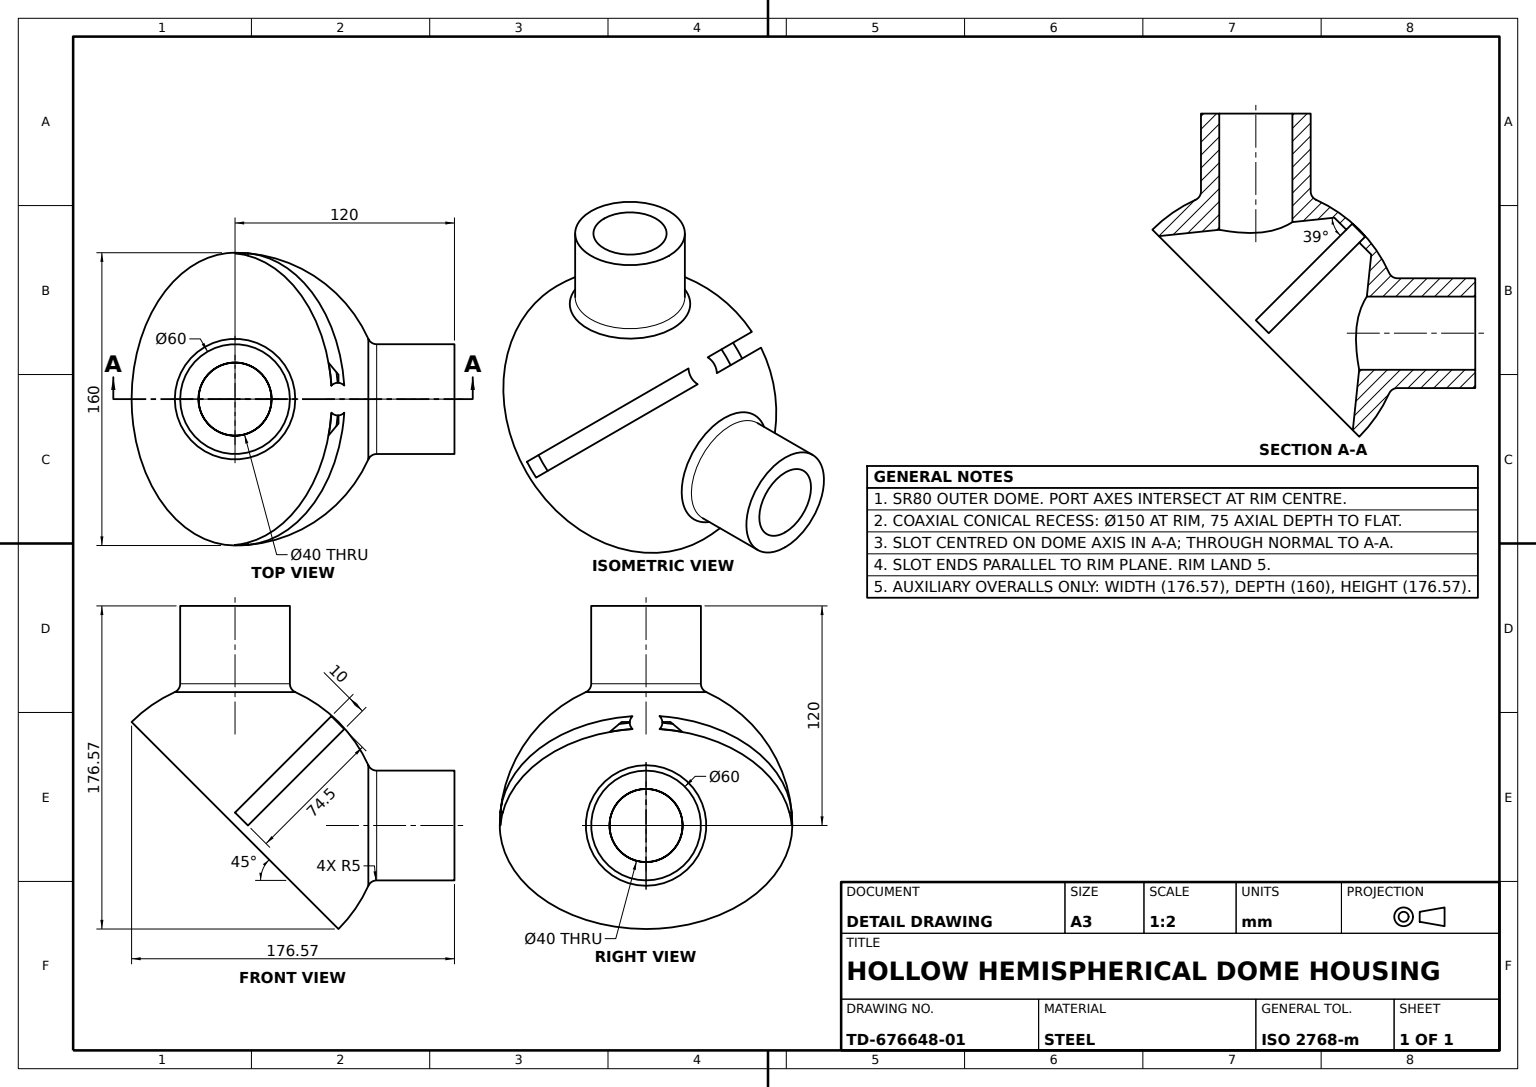
ISO-10303-21;
HEADER;
FILE_DESCRIPTION((''),'2;1');
FILE_NAME('','',(''),(''),'','','');
FILE_SCHEMA(('AUTOMOTIVE_DESIGN'));
ENDSEC;
DATA;
#1=APPLICATION_CONTEXT('');
#2=PRODUCT_CONTEXT('',#1,'mechanical');
#3=PRODUCT('','','',(#2));
#4=PRODUCT_DEFINITION_FORMATION('','',#3);
#5=PRODUCT_DEFINITION_CONTEXT('',#1,'design');
#6=PRODUCT_DEFINITION('','',#4,#5);
#7=PRODUCT_DEFINITION_SHAPE('','',#6);
#8=(LENGTH_UNIT()NAMED_UNIT(*)SI_UNIT(.MILLI.,.METRE.));
#9=(NAMED_UNIT(*)PLANE_ANGLE_UNIT()SI_UNIT($,.RADIAN.));
#10=(NAMED_UNIT(*)SI_UNIT($,.STERADIAN.)SOLID_ANGLE_UNIT());
#11=UNCERTAINTY_MEASURE_WITH_UNIT(LENGTH_MEASURE(1.E-05),#8,'distance_accuracy_value','');
#12=(GEOMETRIC_REPRESENTATION_CONTEXT(3)GLOBAL_UNCERTAINTY_ASSIGNED_CONTEXT((#11))GLOBAL_UNIT_ASSIGNED_CONTEXT((#8,#9,#10))REPRESENTATION_CONTEXT('',''));
#13=CARTESIAN_POINT('',(8.930286,79.5,0.));
#14=VERTEX_POINT('',#13);
#15=CARTESIAN_POINT('',(7.399324,79.5,5.));
#16=VERTEX_POINT('',#15);
#17=CARTESIAN_POINT('',(0.,79.5,0.));
#18=DIRECTION('',(0.,-1.,0.));
#19=DIRECTION('',(0.,0.,1.));
#20=AXIS2_PLACEMENT_3D('',#17,#18,#19);
#21=CIRCLE('',#20,8.930286);
#22=EDGE_CURVE('',#14,#16,#21,.T.);
#23=ORIENTED_EDGE('',*,*,#22,.T.);
#24=CARTESIAN_POINT('',(-7.399324,79.5,5.));
#25=VERTEX_POINT('',#24);
#26=CARTESIAN_POINT('',(-105.,79.5,5.));
#27=DIRECTION('',(1.,0.,0.));
#28=VECTOR('',#27,1000.);
#29=LINE('',#26,#28);
#30=EDGE_CURVE('',#25,#16,#29,.T.);
#31=ORIENTED_EDGE('',*,*,#30,.F.);
#32=CARTESIAN_POINT('',(-8.930286,79.5,0.));
#33=VERTEX_POINT('',#32);
#34=EDGE_CURVE('',#25,#33,#21,.T.);
#35=ORIENTED_EDGE('',*,*,#34,.T.);
#36=CARTESIAN_POINT('',(-7.399324,79.5,-5.));
#37=VERTEX_POINT('',#36);
#38=EDGE_CURVE('',#33,#37,#21,.T.);
#39=ORIENTED_EDGE('',*,*,#38,.T.);
#40=CARTESIAN_POINT('',(7.399324,79.5,-5.));
#41=VERTEX_POINT('',#40);
#42=CARTESIAN_POINT('',(-105.,79.5,-5.));
#43=LINE('',#42,#28);
#44=EDGE_CURVE('',#37,#41,#43,.T.);
#45=ORIENTED_EDGE('',*,*,#44,.T.);
#46=EDGE_CURVE('',#41,#14,#21,.T.);
#47=ORIENTED_EDGE('',*,*,#46,.T.);
#48=EDGE_LOOP('',(#23,#31,#35,#39,#45,#47));
#49=FACE_OUTER_BOUND('',#48,.T.);
#50=DIRECTION('',(0.,1.,0.));
#51=AXIS2_PLACEMENT_3D('',#42,#50,#19);
#52=PLANE('',#51);
#53=ADVANCED_FACE('',(#49),#52,.F.);
#54=CARTESIAN_POINT('',(0.,98.994949,-70.710678));
#55=VERTEX_POINT('',#54);
#56=CARTESIAN_POINT('',(0.,70.710678,-98.994949));
#57=VERTEX_POINT('',#56);
#58=CARTESIAN_POINT('',(0.,84.852814,-84.852814));
#59=DIRECTION('',(0.,0.707106781,-0.707106781));
#60=DIRECTION('',(0.,0.707106781,0.707106781));
#61=AXIS2_PLACEMENT_3D('',#58,#59,#60);
#62=CIRCLE('',#61,20.);
#63=EDGE_CURVE('',#55,#57,#62,.T.);
#64=ORIENTED_EDGE('',*,*,#63,.F.);
#65=EDGE_CURVE('',#57,#55,#62,.T.);
#66=ORIENTED_EDGE('',*,*,#65,.F.);
#67=EDGE_LOOP('',(#64,#66));
#68=FACE_BOUND('',#67,.T.);
#69=CARTESIAN_POINT('',(0.,106.066017,-63.63961));
#70=VERTEX_POINT('',#69);
#71=CARTESIAN_POINT('',(0.,63.63961,-106.066017));
#72=VERTEX_POINT('',#71);
#73=DIRECTION('',(0.,-0.707106781,0.707106781));
#74=DIRECTION('',(0.,-0.707106781,-0.707106781));
#75=AXIS2_PLACEMENT_3D('',#58,#73,#74);
#76=CIRCLE('',#75,30.);
#77=EDGE_CURVE('',#70,#72,#76,.T.);
#78=ORIENTED_EDGE('',*,*,#77,.F.);
#79=EDGE_CURVE('',#72,#70,#76,.T.);
#80=ORIENTED_EDGE('',*,*,#79,.F.);
#81=EDGE_LOOP('',(#78,#80));
#82=FACE_OUTER_BOUND('',#81,.T.);
#83=PLANE('',#61);
#84=ADVANCED_FACE('',(#68,#82),#83,.T.);
#85=CARTESIAN_POINT('',(0.,0.,-75.));
#86=VERTEX_POINT('',#85);
#87=CARTESIAN_POINT('',(0.,0.,75.));
#88=VERTEX_POINT('',#87);
#89=CARTESIAN_POINT('',(0.,0.,0.));
#90=DIRECTION('',(0.,0.,-1.));
#91=AXIS2_PLACEMENT_3D('',#89,#18,#90);
#92=CIRCLE('',#91,75.);
#93=EDGE_CURVE('',#86,#88,#92,.T.);
#94=ORIENTED_EDGE('',*,*,#93,.F.);
#95=EDGE_CURVE('',#88,#86,#92,.T.);
#96=ORIENTED_EDGE('',*,*,#95,.F.);
#97=EDGE_LOOP('',(#94,#96));
#98=FACE_BOUND('',#97,.T.);
#99=CARTESIAN_POINT('',(-80.,0.,0.));
#100=VERTEX_POINT('',#99);
#101=CARTESIAN_POINT('',(80.,0.,0.));
#102=VERTEX_POINT('',#101);
#103=CIRCLE('',#91,80.);
#104=EDGE_CURVE('',#100,#102,#103,.T.);
#105=ORIENTED_EDGE('',*,*,#104,.T.);
#106=EDGE_CURVE('',#102,#100,#103,.T.);
#107=ORIENTED_EDGE('',*,*,#106,.T.);
#108=EDGE_LOOP('',(#105,#107));
#109=FACE_OUTER_BOUND('',#108,.T.);
#110=PLANE('',#91);
#111=ADVANCED_FACE('',(#98,#109),#110,.T.);
#112=CARTESIAN_POINT('',(70.774683,5.,5.));
#113=VERTEX_POINT('',#112);
#114=CARTESIAN_POINT('',(79.686887,5.,5.));
#115=VERTEX_POINT('',#114);
#116=CARTESIAN_POINT('',(-105.,5.,5.));
#117=LINE('',#116,#28);
#118=EDGE_CURVE('',#113,#115,#117,.T.);
#119=ORIENTED_EDGE('',*,*,#118,.T.);
#120=CARTESIAN_POINT('',(79.843597,5.,0.));
#121=VERTEX_POINT('',#120);
#122=CARTESIAN_POINT('',(0.,5.,0.));
#123=AXIS2_PLACEMENT_3D('',#122,#50,#90);
#124=CIRCLE('',#123,79.843597);
#125=EDGE_CURVE('',#115,#121,#124,.T.);
#126=ORIENTED_EDGE('',*,*,#125,.T.);
#127=CARTESIAN_POINT('',(79.686887,5.,-5.));
#128=VERTEX_POINT('',#127);
#129=EDGE_CURVE('',#121,#128,#124,.T.);
#130=ORIENTED_EDGE('',*,*,#129,.T.);
#131=CARTESIAN_POINT('',(70.774683,5.,-5.));
#132=VERTEX_POINT('',#131);
#133=CARTESIAN_POINT('',(-105.,5.,-5.));
#134=LINE('',#133,#28);
#135=EDGE_CURVE('',#132,#128,#134,.T.);
#136=ORIENTED_EDGE('',*,*,#135,.F.);
#137=AXIS2_PLACEMENT_3D('',#122,#18,#90);
#138=CIRCLE('',#137,70.95108);
#139=EDGE_CURVE('',#132,#113,#138,.T.);
#140=ORIENTED_EDGE('',*,*,#139,.T.);
#141=EDGE_LOOP('',(#119,#126,#130,#136,#140));
#142=FACE_OUTER_BOUND('',#141,.T.);
#143=AXIS2_PLACEMENT_3D('',#116,#18,#90);
#144=PLANE('',#143);
#145=ADVANCED_FACE('',(#142),#144,.F.);
#146=CARTESIAN_POINT('',(0.,106.066017,63.63961));
#147=VERTEX_POINT('',#146);
#148=CARTESIAN_POINT('',(0.,75.985459,33.559052));
#149=VERTEX_POINT('',#148);
#150=CARTESIAN_POINT('',(0.,68.907495,26.481088));
#151=VECTOR('',#74,1000.);
#152=LINE('',#150,#151);
#153=EDGE_CURVE('',#147,#149,#152,.T.);
#154=ORIENTED_EDGE('',*,*,#153,.F.);
#155=CARTESIAN_POINT('',(0.,63.63961,106.066017));
#156=VERTEX_POINT('',#155);
#157=CARTESIAN_POINT('',(0.,84.852814,84.852814));
#158=AXIS2_PLACEMENT_3D('',#157,#60,#73);
#159=CIRCLE('',#158,30.);
#160=EDGE_CURVE('',#156,#147,#159,.T.);
#161=ORIENTED_EDGE('',*,*,#160,.F.);
#162=CARTESIAN_POINT('',(0.,33.559052,75.985459));
#163=VERTEX_POINT('',#162);
#164=CARTESIAN_POINT('',(0.,26.481088,68.907495));
#165=LINE('',#164,#151);
#166=EDGE_CURVE('',#156,#163,#165,.T.);
#167=ORIENTED_EDGE('',*,*,#166,.T.);
#168=CARTESIAN_POINT('',(0.,54.772256,54.772256));
#169=AXIS2_PLACEMENT_3D('',#168,#60,#59);
#170=CIRCLE('',#169,30.);
#171=EDGE_CURVE('',#163,#149,#170,.T.);
#172=ORIENTED_EDGE('',*,*,#171,.T.);
#173=EDGE_LOOP('',(#154,#161,#167,#172));
#174=FACE_OUTER_BOUND('',#173,.T.);
#175=CARTESIAN_POINT('',(0.,47.694291,47.694291));
#176=AXIS2_PLACEMENT_3D('',#175,#74,#73);
#177=CYLINDRICAL_SURFACE('',#176,30.);
#178=ADVANCED_FACE('',(#174),#177,.T.);
#179=CARTESIAN_POINT('',(0.,28.257429,74.843288));
#180=VERTEX_POINT('',#179);
#181=CARTESIAN_POINT('',(0.,30.023518,79.520993));
#182=AXIS2_PLACEMENT_3D('',#181,#27,#90);
#183=CIRCLE('',#182,5.);
#184=EDGE_CURVE('',#180,#163,#183,.T.);
#185=ORIENTED_EDGE('',*,*,#184,.T.);
#186=EDGE_CURVE('',#149,#163,#170,.T.);
#187=ORIENTED_EDGE('',*,*,#186,.F.);
#188=CARTESIAN_POINT('',(0.,74.843288,28.257429));
#189=VERTEX_POINT('',#188);
#190=CARTESIAN_POINT('',(0.,79.520993,30.023518));
#191=DIRECTION('',(-1.,0.,0.));
#192=AXIS2_PLACEMENT_3D('',#190,#191,#19);
#193=CIRCLE('',#192,5.);
#194=EDGE_CURVE('',#189,#149,#193,.T.);
#195=ORIENTED_EDGE('',*,*,#194,.F.);
#196=CARTESIAN_POINT('',(0.,51.550358,51.550358));
#197=AXIS2_PLACEMENT_3D('',#196,#74,#59);
#198=CIRCLE('',#197,32.941176);
#199=EDGE_CURVE('',#180,#189,#198,.T.);
#200=ORIENTED_EDGE('',*,*,#199,.F.);
#201=EDGE_LOOP('',(#185,#187,#195,#200));
#202=FACE_OUTER_BOUND('',#201,.T.);
#203=AXIS2_PLACEMENT_3D('',#168,#74,#59);
#204=TOROIDAL_SURFACE('',#203,35.,5.);
#205=ADVANCED_FACE('',(#202),#204,.F.);
#206=CARTESIAN_POINT('',(0.,98.994949,70.710678));
#207=VERTEX_POINT('',#206);
#208=CARTESIAN_POINT('',(0.,70.710678,98.994949));
#209=VERTEX_POINT('',#208);
#210=AXIS2_PLACEMENT_3D('',#157,#74,#59);
#211=CIRCLE('',#210,20.);
#212=EDGE_CURVE('',#207,#209,#211,.T.);
#213=ORIENTED_EDGE('',*,*,#212,.F.);
#214=CARTESIAN_POINT('',(0.,57.069943,28.785672));
#215=VERTEX_POINT('',#214);
#216=CARTESIAN_POINT('',(0.,45.961941,17.67767));
#217=VECTOR('',#60,1000.);
#218=LINE('',#216,#217);
#219=EDGE_CURVE('',#215,#207,#218,.T.);
#220=ORIENTED_EDGE('',*,*,#219,.F.);
#221=CARTESIAN_POINT('',(0.,25.812875,54.097146));
#222=VERTEX_POINT('',#221);
#223=CARTESIAN_POINT('',(1.321111,57.069943,28.785672));
#224=CARTESIAN_POINT('',(2.628522,56.918047,28.817066));
#225=CARTESIAN_POINT('',(4.246145,56.545365,28.901953));
#226=CARTESIAN_POINT('',(4.56981,56.461343,28.921355));
#227=CARTESIAN_POINT('',(5.209011,56.276916,28.964836));
#228=CARTESIAN_POINT('',(5.524817,56.176517,28.988912));
#229=CARTESIAN_POINT('',(6.461346,55.852019,29.06855));
#230=CARTESIAN_POINT('',(7.071206,55.604675,29.131485));
#231=CARTESIAN_POINT('',(8.263837,55.053183,29.280102));
#232=CARTESIAN_POINT('',(8.846605,54.74903,29.365783));
#233=CARTESIAN_POINT('',(9.986057,54.087397,29.564114));
#234=CARTESIAN_POINT('',(10.539799,53.731357,29.676411));
#235=CARTESIAN_POINT('',(12.134798,52.609,30.053427));
#236=CARTESIAN_POINT('',(13.119705,51.783991,30.359429));
#237=CARTESIAN_POINT('',(14.48557,50.448177,30.925042));
#238=CARTESIAN_POINT('',(14.923117,49.984812,31.132268));
#239=CARTESIAN_POINT('',(15.743946,49.044679,31.578323));
#240=CARTESIAN_POINT('',(16.129389,48.565996,31.817888));
#241=CARTESIAN_POINT('',(17.212018,47.106939,32.589816));
#242=CARTESIAN_POINT('',(17.83638,46.104015,33.175112));
#243=CARTESIAN_POINT('',(18.616197,44.556841,34.177448));
#244=CARTESIAN_POINT('',(18.84657,44.039831,34.528624));
#245=CARTESIAN_POINT('',(19.244435,43.013834,35.258002));
#246=CARTESIAN_POINT('',(19.412759,42.503204,35.637259));
#247=CARTESIAN_POINT('',(19.687945,41.486443,36.424695));
#248=CARTESIAN_POINT('',(19.79481,40.980311,36.832872));
#249=CARTESIAN_POINT('',(19.945033,39.971974,37.678162));
#250=CARTESIAN_POINT('',(19.988273,39.466756,38.118079));
#251=CARTESIAN_POINT('',(20.017146,37.986493,39.453391));
#252=CARTESIAN_POINT('',(19.905318,37.042308,40.367012));
#253=CARTESIAN_POINT('',(19.543234,35.679289,41.761911));
#254=CARTESIAN_POINT('',(19.389181,35.232214,42.232773));
#255=CARTESIAN_POINT('',(19.016593,34.362194,43.172806));
#256=CARTESIAN_POINT('',(18.799907,33.942827,43.637984));
#257=CARTESIAN_POINT('',(18.061557,32.727049,45.016752));
#258=CARTESIAN_POINT('',(17.452481,31.972569,45.913773));
#259=CARTESIAN_POINT('',(16.358643,30.914885,47.214376));
#260=CARTESIAN_POINT('',(15.967324,30.578446,47.635873));
#261=CARTESIAN_POINT('',(15.139651,29.941022,48.446388));
#262=CARTESIAN_POINT('',(14.702254,29.639028,48.836658));
#263=CARTESIAN_POINT('',(13.780613,29.066497,49.586025));
#264=CARTESIAN_POINT('',(13.29637,28.795965,49.945125));
#265=CARTESIAN_POINT('',(12.279891,28.285505,50.630135));
#266=CARTESIAN_POINT('',(11.745496,28.044946,50.956943));
#267=CARTESIAN_POINT('',(10.103299,27.382989,51.864381));
#268=CARTESIAN_POINT('',(8.947754,27.015308,52.379734));
#269=CARTESIAN_POINT('',(7.123273,26.567464,53.013403));
#270=CARTESIAN_POINT('',(6.497772,26.435263,53.201767));
#271=CARTESIAN_POINT('',(5.223722,26.208052,53.526788));
#272=CARTESIAN_POINT('',(4.581881,26.1141,53.661919));
#273=CARTESIAN_POINT('',(2.642329,25.888634,53.986939));
#274=CARTESIAN_POINT('',(1.33072,25.812875,54.097146));
#275=B_SPLINE_CURVE_WITH_KNOTS('',3,(#214,#223,#224,#225,#226,#227,#228,#229,#230,#231,#232,#233,#234,#235,#236,#237,#238,#239,#240,#241,#242,#243,#244,#245,#246,#247,#248,#249,#250,#251,#252,#253,#254,#255,#256,#257,#258,#259,#260,#261,#262,#263,#264,#265,#266,#267,#268,#269,#270,#271,#272,#273,#274,#221),.UNSPECIFIED.,.F.,.F.,(4,2,2,2,2,2,2,2,2,2,2,2,2,2,2,2,2,2,2,2,2,2,2,2,2,2,4),(0.022902913,0.026848629,0.027835058,0.028821487,0.030794345,0.032767203,0.034740061,0.038685777,0.040658635,0.042631493,0.046577209,0.048550066,0.050522924,0.052495782,0.05446864,0.058414356,0.060387214,0.062360072,0.066305788,0.068278646,0.070251504,0.072224362,0.07419722,0.078142935,0.080115793,0.082088651,0.086034367),.UNSPECIFIED.);
#276=EDGE_CURVE('',#215,#222,#275,.T.);
#277=ORIENTED_EDGE('',*,*,#276,.T.);
#278=CARTESIAN_POINT('',(0.,17.67767,45.961941));
#279=LINE('',#278,#217);
#280=EDGE_CURVE('',#222,#209,#279,.T.);
#281=ORIENTED_EDGE('',*,*,#280,.T.);
#282=EDGE_LOOP('',(#213,#220,#277,#281));
#283=FACE_OUTER_BOUND('',#282,.T.);
#284=CARTESIAN_POINT('',(0.,31.819805,31.819805));
#285=AXIS2_PLACEMENT_3D('',#284,#60,#73);
#286=CYLINDRICAL_SURFACE('',#285,20.);
#287=ADVANCED_FACE('',(#283),#286,.F.);
#288=CARTESIAN_POINT('',(0.,80.,0.));
#289=VERTEX_POINT('',#288);
#290=AXIS2_PLACEMENT_3D('',#89,#19,#27);
#291=CIRCLE('',#290,80.);
#292=EDGE_CURVE('',#289,#33,#291,.T.);
#293=ORIENTED_EDGE('',*,*,#292,.F.);
#294=AXIS2_PLACEMENT_3D('',#89,#90,#191);
#295=CIRCLE('',#294,80.);
#296=EDGE_CURVE('',#289,#14,#295,.T.);
#297=ORIENTED_EDGE('',*,*,#296,.T.);
#298=ORIENTED_EDGE('',*,*,#46,.F.);
#299=CARTESIAN_POINT('',(0.,0.,-5.));
#300=AXIS2_PLACEMENT_3D('',#299,#19,#191);
#301=CIRCLE('',#300,79.843597);
#302=EDGE_CURVE('',#128,#41,#301,.T.);
#303=ORIENTED_EDGE('',*,*,#302,.F.);
#304=ORIENTED_EDGE('',*,*,#129,.F.);
#305=EDGE_CURVE('',#121,#102,#295,.T.);
#306=ORIENTED_EDGE('',*,*,#305,.T.);
#307=ORIENTED_EDGE('',*,*,#104,.F.);
#308=CARTESIAN_POINT('',(-79.843597,5.,0.));
#309=VERTEX_POINT('',#308);
#310=EDGE_CURVE('',#309,#100,#291,.T.);
#311=ORIENTED_EDGE('',*,*,#310,.F.);
#312=CARTESIAN_POINT('',(-79.686887,5.,-5.));
#313=VERTEX_POINT('',#312);
#314=EDGE_CURVE('',#313,#309,#124,.T.);
#315=ORIENTED_EDGE('',*,*,#314,.F.);
#316=EDGE_CURVE('',#37,#313,#301,.T.);
#317=ORIENTED_EDGE('',*,*,#316,.F.);
#318=ORIENTED_EDGE('',*,*,#38,.F.);
#319=EDGE_LOOP('',(#293,#297,#298,#303,#304,#306,#307,#311,#315,#317,#318));
#320=FACE_OUTER_BOUND('',#319,.T.);
#321=CARTESIAN_POINT('',(0.,74.843288,-28.257429));
#322=VERTEX_POINT('',#321);
#323=CARTESIAN_POINT('',(0.,28.257429,-74.843288));
#324=VERTEX_POINT('',#323);
#325=CARTESIAN_POINT('',(0.,51.550358,-51.550358));
#326=AXIS2_PLACEMENT_3D('',#325,#73,#74);
#327=CIRCLE('',#326,32.941176);
#328=EDGE_CURVE('',#322,#324,#327,.T.);
#329=ORIENTED_EDGE('',*,*,#328,.T.);
#330=EDGE_CURVE('',#324,#322,#327,.T.);
#331=ORIENTED_EDGE('',*,*,#330,.T.);
#332=EDGE_LOOP('',(#329,#331));
#333=FACE_BOUND('',#332,.T.);
#334=SPHERICAL_SURFACE('',#290,80.);
#335=ADVANCED_FACE('',(#320,#333),#334,.T.);
#336=ORIENTED_EDGE('',*,*,#77,.T.);
#337=CARTESIAN_POINT('',(0.,33.559052,-75.985459));
#338=VERTEX_POINT('',#337);
#339=CARTESIAN_POINT('',(0.,26.481088,-68.907495));
#340=VECTOR('',#73,1000.);
#341=LINE('',#339,#340);
#342=EDGE_CURVE('',#72,#338,#341,.T.);
#343=ORIENTED_EDGE('',*,*,#342,.T.);
#344=CARTESIAN_POINT('',(0.,75.985459,-33.559052));
#345=VERTEX_POINT('',#344);
#346=CARTESIAN_POINT('',(0.,54.772256,-54.772256));
#347=AXIS2_PLACEMENT_3D('',#346,#59,#74);
#348=CIRCLE('',#347,30.);
#349=EDGE_CURVE('',#338,#345,#348,.T.);
#350=ORIENTED_EDGE('',*,*,#349,.T.);
#351=CARTESIAN_POINT('',(0.,68.907495,-26.481088));
#352=LINE('',#351,#340);
#353=EDGE_CURVE('',#70,#345,#352,.T.);
#354=ORIENTED_EDGE('',*,*,#353,.F.);
#355=EDGE_LOOP('',(#336,#343,#350,#354));
#356=FACE_OUTER_BOUND('',#355,.T.);
#357=CARTESIAN_POINT('',(0.,47.694291,-47.694291));
#358=AXIS2_PLACEMENT_3D('',#357,#73,#74);
#359=CYLINDRICAL_SURFACE('',#358,30.);
#360=ADVANCED_FACE('',(#356),#359,.T.);
#361=CARTESIAN_POINT('',(0.,79.520993,-30.023518));
#362=AXIS2_PLACEMENT_3D('',#361,#27,#90);
#363=CIRCLE('',#362,5.);
#364=EDGE_CURVE('',#322,#345,#363,.T.);
#365=ORIENTED_EDGE('',*,*,#364,.T.);
#366=ORIENTED_EDGE('',*,*,#349,.F.);
#367=CARTESIAN_POINT('',(0.,30.023518,-79.520993));
#368=AXIS2_PLACEMENT_3D('',#367,#191,#19);
#369=CIRCLE('',#368,5.);
#370=EDGE_CURVE('',#324,#338,#369,.T.);
#371=ORIENTED_EDGE('',*,*,#370,.F.);
#372=ORIENTED_EDGE('',*,*,#328,.F.);
#373=EDGE_LOOP('',(#365,#366,#371,#372));
#374=FACE_OUTER_BOUND('',#373,.T.);
#375=AXIS2_PLACEMENT_3D('',#346,#73,#74);
#376=TOROIDAL_SURFACE('',#375,35.,5.);
#377=ADVANCED_FACE('',(#374),#376,.F.);
#378=EDGE_CURVE('',#189,#180,#198,.T.);
#379=ORIENTED_EDGE('',*,*,#378,.F.);
#380=ORIENTED_EDGE('',*,*,#194,.T.);
#381=ORIENTED_EDGE('',*,*,#171,.F.);
#382=ORIENTED_EDGE('',*,*,#184,.F.);
#383=EDGE_LOOP('',(#379,#380,#381,#382));
#384=FACE_OUTER_BOUND('',#383,.T.);
#385=ADVANCED_FACE('',(#384),#204,.F.);
#386=ORIENTED_EDGE('',*,*,#63,.T.);
#387=CARTESIAN_POINT('',(0.,25.812875,-54.097146));
#388=VERTEX_POINT('',#387);
#389=CARTESIAN_POINT('',(0.,17.67767,-45.961941));
#390=VECTOR('',#59,1000.);
#391=LINE('',#389,#390);
#392=EDGE_CURVE('',#388,#57,#391,.T.);
#393=ORIENTED_EDGE('',*,*,#392,.F.);
#394=CARTESIAN_POINT('',(0.,57.069943,-28.785672));
#395=VERTEX_POINT('',#394);
#396=CARTESIAN_POINT('',(1.335921,57.069943,-28.785672));
#397=CARTESIAN_POINT('',(2.645466,56.914763,-28.817797));
#398=CARTESIAN_POINT('',(4.573353,56.469667,-28.919204));
#399=CARTESIAN_POINT('',(5.211424,56.285227,-28.962225));
#400=CARTESIAN_POINT('',(6.468901,55.849278,-29.06923));
#401=CARTESIAN_POINT('',(7.080753,55.60063,-29.132534));
#402=CARTESIAN_POINT('',(8.273496,55.04834,-29.281447));
#403=CARTESIAN_POINT('',(8.854381,54.744685,-29.367058));
#404=CARTESIAN_POINT('',(9.986857,54.08676,-29.564333));
#405=CARTESIAN_POINT('',(10.54024,53.731202,-29.676429));
#406=CARTESIAN_POINT('',(12.14503,52.601487,-30.056019));
#407=CARTESIAN_POINT('',(13.128972,51.775315,-30.362983));
#408=CARTESIAN_POINT('',(14.486638,50.446938,-30.925627));
#409=CARTESIAN_POINT('',(14.919282,49.989095,-31.130273));
#410=CARTESIAN_POINT('',(15.744169,49.044534,-31.578355));
#411=CARTESIAN_POINT('',(16.134274,48.559874,-31.820973));
#412=CARTESIAN_POINT('',(17.2206,47.09444,-32.596741));
#413=CARTESIAN_POINT('',(17.84135,46.094018,-33.181625));
#414=CARTESIAN_POINT('',(18.613037,44.563178,-34.173325));
#415=CARTESIAN_POINT('',(18.844233,44.045797,-34.524395));
#416=CARTESIAN_POINT('',(19.246305,43.009072,-35.261375));
#417=CARTESIAN_POINT('',(19.415272,42.495244,-35.643232));
#418=CARTESIAN_POINT('',(19.82789,40.96669,-36.82761));
#419=CARTESIAN_POINT('',(19.978176,39.964981,-37.66882));
#420=CARTESIAN_POINT('',(20.002723,38.730727,-38.781989));
#421=CARTESIAN_POINT('',(19.999336,38.484019,-39.00842));
#422=CARTESIAN_POINT('',(19.975897,37.997015,-39.462951));
#423=CARTESIAN_POINT('',(19.95591,37.756576,-39.691153));
#424=CARTESIAN_POINT('',(19.871586,37.043969,-40.378209));
#425=CARTESIAN_POINT('',(19.782947,36.580495,-40.83951));
#426=CARTESIAN_POINT('',(19.541685,35.674639,-41.766789));
#427=CARTESIAN_POINT('',(19.389062,35.232259,-42.232769));
#428=CARTESIAN_POINT('',(19.018787,34.366997,-43.167572));
#429=CARTESIAN_POINT('',(18.799703,33.942197,-43.638649));
#430=CARTESIAN_POINT('',(18.056783,32.71978,-45.025093));
#431=CARTESIAN_POINT('',(17.446827,31.967173,-45.920421));
#432=CARTESIAN_POINT('',(16.362173,30.918263,-47.210217));
#433=CARTESIAN_POINT('',(15.97023,30.580666,-47.633047));
#434=CARTESIAN_POINT('',(15.136103,29.938307,-48.449844));
#435=CARTESIAN_POINT('',(14.696597,29.635243,-48.841567));
#436=CARTESIAN_POINT('',(13.31253,28.776267,-49.965988));
#437=CARTESIAN_POINT('',(12.303075,28.270036,-50.648421));
#438=CARTESIAN_POINT('',(10.928706,27.715622,-51.408384));
#439=CARTESIAN_POINT('',(10.647866,27.608637,-51.555778));
#440=CARTESIAN_POINT('',(10.081022,27.40485,-51.83773));
#441=CARTESIAN_POINT('',(9.794273,27.30773,-51.97272));
#442=CARTESIAN_POINT('',(8.924187,27.030265,-52.359833));
#443=CARTESIAN_POINT('',(8.331035,26.863774,-52.594134));
#444=CARTESIAN_POINT('',(7.118712,26.566498,-53.014779));
#445=CARTESIAN_POINT('',(6.499542,26.435714,-53.201126));
#446=CARTESIAN_POINT('',(5.234596,26.209857,-53.524201));
#447=CARTESIAN_POINT('',(4.585015,26.114435,-53.661435));
#448=CARTESIAN_POINT('',(2.631783,25.887465,-53.988624));
#449=CARTESIAN_POINT('',(1.320422,25.812875,-54.097146));
#450=B_SPLINE_CURVE_WITH_KNOTS('',3,(#394,#396,#397,#398,#399,#400,#401,#402,#403,#404,#405,#406,#407,#408,#409,#410,#411,#412,#413,#414,#415,#416,#417,#418,#419,#420,#421,#422,#423,#424,#425,#426,#427,#428,#429,#430,#431,#432,#433,#434,#435,#436,#437,#438,#439,#440,#441,#442,#443,#444,#445,#446,#447,#448,#449,#387),.UNSPECIFIED.,.F.,.F.,(4,2,2,2,2,2,2,2,2,2,2,2,2,2,2,2,2,2,2,2,2,2,2,2,2,2,2,4),(0.054053573,0.058000914,0.059974585,0.061948255,0.063921926,0.065895597,0.069842938,0.071816608,0.073790279,0.07773762,0.079711291,0.081684962,0.085632303,0.086619138,0.087605973,0.089579644,0.091553315,0.093526985,0.097474326,0.099447997,0.101421668,0.105369009,0.106355844,0.10734268,0.10931635,0.111290021,0.113263691,0.117211033),.UNSPECIFIED.);
#451=EDGE_CURVE('',#395,#388,#450,.T.);
#452=ORIENTED_EDGE('',*,*,#451,.F.);
#453=CARTESIAN_POINT('',(0.,45.961941,-17.67767));
#454=LINE('',#453,#390);
#455=EDGE_CURVE('',#395,#55,#454,.T.);
#456=ORIENTED_EDGE('',*,*,#455,.T.);
#457=EDGE_LOOP('',(#386,#393,#452,#456));
#458=FACE_OUTER_BOUND('',#457,.T.);
#459=CARTESIAN_POINT('',(0.,31.819805,-31.819805));
#460=AXIS2_PLACEMENT_3D('',#459,#59,#60);
#461=CYLINDRICAL_SURFACE('',#460,20.);
#462=ADVANCED_FACE('',(#458),#461,.F.);
#463=ORIENTED_EDGE('',*,*,#455,.F.);
#464=CARTESIAN_POINT('',(-0.661116,25.812875,-54.097146));
#465=CARTESIAN_POINT('',(-1.324519,25.831735,-54.069771));
#466=CARTESIAN_POINT('',(-2.656067,25.908663,-53.958369));
#467=CARTESIAN_POINT('',(-3.312478,25.966064,-53.875311));
#468=CARTESIAN_POINT('',(-5.253168,26.193105,-53.548046));
#469=CARTESIAN_POINT('',(-6.509911,26.416994,-53.226313));
#470=CARTESIAN_POINT('',(-8.339375,26.865929,-52.591092));
#471=CARTESIAN_POINT('',(-8.943219,27.035775,-52.352096));
#472=CARTESIAN_POINT('',(-10.108673,27.408571,-51.832082));
#473=CARTESIAN_POINT('',(-10.671598,27.611557,-51.55099));
#474=CARTESIAN_POINT('',(-12.302751,28.270614,-50.647712));
#475=CARTESIAN_POINT('',(-13.313931,28.776129,-49.966001));
#476=CARTESIAN_POINT('',(-14.712997,29.645934,-48.827657));
#477=CARTESIAN_POINT('',(-15.153733,29.95113,-48.433403));
#478=CARTESIAN_POINT('',(-15.979849,30.588854,-47.622776));
#479=CARTESIAN_POINT('',(-16.366227,30.922,-47.205587));
#480=CARTESIAN_POINT('',(-17.086085,31.618504,-46.349198));
#481=CARTESIAN_POINT('',(-17.419569,31.981856,-45.909994));
#482=CARTESIAN_POINT('',(-18.032481,32.741488,-45.010759));
#483=CARTESIAN_POINT('',(-18.312707,33.139637,-44.548691));
#484=CARTESIAN_POINT('',(-19.052992,34.361511,-43.163495));
#485=CARTESIAN_POINT('',(-19.420158,35.2188,-42.233453));
#486=CARTESIAN_POINT('',(-19.782926,36.580188,-40.839802));
#487=CARTESIAN_POINT('',(-19.872449,37.048073,-40.37409));
#488=CARTESIAN_POINT('',(-19.98503,38.005912,-39.450922));
#489=CARTESIAN_POINT('',(-20.007615,38.490066,-38.998991));
#490=CARTESIAN_POINT('',(-19.978067,39.959818,-37.673578));
#491=CARTESIAN_POINT('',(-19.82953,40.962711,-36.83039));
#492=CARTESIAN_POINT('',(-19.481242,42.250322,-35.833083));
#493=CARTESIAN_POINT('',(-19.403208,42.509931,-35.636199));
#494=CARTESIAN_POINT('',(-19.232579,43.02658,-35.252718));
#495=CARTESIAN_POINT('',(-19.139819,43.284328,-35.065557));
#496=CARTESIAN_POINT('',(-18.839757,44.05591,-34.517509));
#497=CARTESIAN_POINT('',(-18.610731,44.568101,-34.170042));
#498=CARTESIAN_POINT('',(-18.096277,45.587954,-33.509555));
#499=CARTESIAN_POINT('',(-17.810849,46.09562,-33.196538));
#500=CARTESIAN_POINT('',(-17.183399,47.105621,-32.603878));
#501=CARTESIAN_POINT('',(-16.840176,47.60916,-32.323747));
#502=CARTESIAN_POINT('',(-15.746628,49.079596,-31.546913));
#503=CARTESIAN_POINT('',(-14.927706,50.01693,-31.107282));
#504=CARTESIAN_POINT('',(-13.564452,51.348438,-30.544035));
#505=CARTESIAN_POINT('',(-13.084987,51.781626,-30.371688));
#506=CARTESIAN_POINT('',(-12.090294,52.609273,-30.060021));
#507=CARTESIAN_POINT('',(-11.576734,53.002702,-29.920959));
#508=CARTESIAN_POINT('',(-9.98676,54.118427,-29.54684));
#509=CARTESIAN_POINT('',(-8.861731,54.777111,-29.354454));
#510=CARTESIAN_POINT('',(-7.06264,55.608433,-29.130494));
#511=CARTESIAN_POINT('',(-6.443234,55.858937,-29.066812));
#512=CARTESIAN_POINT('',(-5.196896,56.289478,-28.961231));
#513=CARTESIAN_POINT('',(-4.566154,56.471447,-28.918795));
#514=CARTESIAN_POINT('',(-3.289091,56.76605,-28.851682));
#515=CARTESIAN_POINT('',(-2.64277,56.878684,-28.827002));
#516=CARTESIAN_POINT('',(-1.333776,57.030632,-28.794001));
#517=CARTESIAN_POINT('',(-0.668876,57.069943,-28.785672));
#518=B_SPLINE_CURVE_WITH_KNOTS('',3,(#387,#464,#465,#466,#467,#468,#469,#470,#471,#472,#473,#474,#475,#476,#477,#478,#479,#480,#481,#482,#483,#484,#485,#486,#487,#488,#489,#490,#491,#492,#493,#494,#495,#496,#497,#498,#499,#500,#501,#502,#503,#504,#505,#506,#507,#508,#509,#510,#511,#512,#513,#514,#515,#516,#517,#394),.UNSPECIFIED.,.F.,.F.,(4,2,2,2,2,2,2,2,2,2,2,2,2,2,2,2,2,2,2,2,2,2,2,2,2,2,2,4),(0.117211033,0.119187408,0.121163783,0.125116533,0.127092908,0.129069283,0.133022034,0.134998409,0.136974784,0.138951159,0.140927534,0.144880284,0.146856659,0.148833034,0.152785785,0.153773972,0.15476216,0.156738535,0.15871491,0.160691285,0.164644035,0.16662041,0.168596785,0.172549536,0.174525911,0.176502286,0.178478661,0.180455036),.UNSPECIFIED.);
#519=EDGE_CURVE('',#388,#395,#518,.T.);
#520=ORIENTED_EDGE('',*,*,#519,.F.);
#521=ORIENTED_EDGE('',*,*,#392,.T.);
#522=ORIENTED_EDGE('',*,*,#65,.T.);
#523=EDGE_LOOP('',(#463,#520,#521,#522));
#524=FACE_OUTER_BOUND('',#523,.T.);
#525=ADVANCED_FACE('',(#524),#461,.F.);
#526=ORIENTED_EDGE('',*,*,#296,.F.);
#527=ORIENTED_EDGE('',*,*,#292,.T.);
#528=ORIENTED_EDGE('',*,*,#34,.F.);
#529=CARTESIAN_POINT('',(-79.686887,5.,5.));
#530=VERTEX_POINT('',#529);
#531=CARTESIAN_POINT('',(0.,0.,5.));
#532=AXIS2_PLACEMENT_3D('',#531,#90,#27);
#533=CIRCLE('',#532,79.843597);
#534=EDGE_CURVE('',#530,#25,#533,.T.);
#535=ORIENTED_EDGE('',*,*,#534,.F.);
#536=EDGE_CURVE('',#309,#530,#124,.T.);
#537=ORIENTED_EDGE('',*,*,#536,.F.);
#538=ORIENTED_EDGE('',*,*,#310,.T.);
#539=ORIENTED_EDGE('',*,*,#106,.F.);
#540=ORIENTED_EDGE('',*,*,#305,.F.);
#541=ORIENTED_EDGE('',*,*,#125,.F.);
#542=EDGE_CURVE('',#16,#115,#533,.T.);
#543=ORIENTED_EDGE('',*,*,#542,.F.);
#544=ORIENTED_EDGE('',*,*,#22,.F.);
#545=EDGE_LOOP('',(#526,#527,#528,#535,#537,#538,#539,#540,#541,#543,#544));
#546=FACE_OUTER_BOUND('',#545,.T.);
#547=ORIENTED_EDGE('',*,*,#199,.T.);
#548=ORIENTED_EDGE('',*,*,#378,.T.);
#549=EDGE_LOOP('',(#547,#548));
#550=FACE_BOUND('',#549,.T.);
#551=ADVANCED_FACE('',(#546,#550),#334,.T.);
#552=CARTESIAN_POINT('',(-70.774683,5.,5.));
#553=VERTEX_POINT('',#552);
#554=EDGE_CURVE('',#530,#553,#117,.T.);
#555=ORIENTED_EDGE('',*,*,#554,.T.);
#556=CARTESIAN_POINT('',(-70.774683,5.,-5.));
#557=VERTEX_POINT('',#556);
#558=EDGE_CURVE('',#553,#557,#138,.T.);
#559=ORIENTED_EDGE('',*,*,#558,.T.);
#560=EDGE_CURVE('',#313,#557,#134,.T.);
#561=ORIENTED_EDGE('',*,*,#560,.F.);
#562=ORIENTED_EDGE('',*,*,#314,.T.);
#563=ORIENTED_EDGE('',*,*,#536,.T.);
#564=EDGE_LOOP('',(#555,#559,#561,#562,#563));
#565=FACE_OUTER_BOUND('',#564,.T.);
#566=ADVANCED_FACE('',(#565),#144,.F.);
#567=EDGE_CURVE('',#147,#156,#159,.T.);
#568=ORIENTED_EDGE('',*,*,#567,.F.);
#569=ORIENTED_EDGE('',*,*,#153,.T.);
#570=ORIENTED_EDGE('',*,*,#186,.T.);
#571=ORIENTED_EDGE('',*,*,#166,.F.);
#572=EDGE_LOOP('',(#568,#569,#570,#571));
#573=FACE_OUTER_BOUND('',#572,.T.);
#574=ADVANCED_FACE('',(#573),#177,.T.);
#575=ORIENTED_EDGE('',*,*,#353,.T.);
#576=EDGE_CURVE('',#345,#338,#348,.T.);
#577=ORIENTED_EDGE('',*,*,#576,.T.);
#578=ORIENTED_EDGE('',*,*,#342,.F.);
#579=ORIENTED_EDGE('',*,*,#79,.T.);
#580=EDGE_LOOP('',(#575,#577,#578,#579));
#581=FACE_OUTER_BOUND('',#580,.T.);
#582=ADVANCED_FACE('',(#581),#359,.T.);
#583=EDGE_CURVE('',#209,#207,#211,.T.);
#584=ORIENTED_EDGE('',*,*,#583,.T.);
#585=ORIENTED_EDGE('',*,*,#212,.T.);
#586=EDGE_LOOP('',(#584,#585));
#587=FACE_BOUND('',#586,.T.);
#588=ORIENTED_EDGE('',*,*,#567,.T.);
#589=ORIENTED_EDGE('',*,*,#160,.T.);
#590=EDGE_LOOP('',(#588,#589));
#591=FACE_OUTER_BOUND('',#590,.T.);
#592=AXIS2_PLACEMENT_3D('',#157,#60,#59);
#593=PLANE('',#592);
#594=ADVANCED_FACE('',(#587,#591),#593,.T.);
#595=CARTESIAN_POINT('',(13.361302,75.,5.));
#596=VERTEX_POINT('',#595);
#597=CARTESIAN_POINT('',(0.,75.,14.266198));
#598=VERTEX_POINT('',#597);
#599=CARTESIAN_POINT('',(0.,75.,0.));
#600=AXIS2_PLACEMENT_3D('',#599,#18,#90);
#601=CIRCLE('',#600,14.266198);
#602=EDGE_CURVE('',#596,#598,#601,.T.);
#603=ORIENTED_EDGE('',*,*,#602,.F.);
#604=CARTESIAN_POINT('',(61.264447,16.714965,5.));
#605=CARTESIAN_POINT('',(51.751076,28.427386,5.));
#606=CARTESIAN_POINT('',(37.447215,45.968576,5.));
#607=CARTESIAN_POINT('',(32.674232,51.811651,5.));
#608=CARTESIAN_POINT('',(25.484302,60.551055,5.));
#609=CARTESIAN_POINT('',(23.082601,63.460005,5.));
#610=CARTESIAN_POINT('',(19.460626,67.807365,5.));
#611=CARTESIAN_POINT('',(18.249987,69.253744,5.));
#612=CARTESIAN_POINT('',(15.816891,72.136726,5.));
#613=CARTESIAN_POINT('',(14.594778,73.573401,5.));
#614=B_SPLINE_CURVE_WITH_KNOTS('',3,(#112,#604,#605,#606,#607,#608,#609,#610,#611,#612,#613,#595),.UNSPECIFIED.,.F.,.F.,(4,2,2,2,2,4),(0.127857249,0.173124952,0.195758804,0.20707573,0.212734193,0.218392656),.UNSPECIFIED.);
#615=EDGE_CURVE('',#113,#596,#614,.T.);
#616=ORIENTED_EDGE('',*,*,#615,.F.);
#617=ORIENTED_EDGE('',*,*,#139,.F.);
#618=CARTESIAN_POINT('',(13.361302,75.,-5.));
#619=VERTEX_POINT('',#618);
#620=CARTESIAN_POINT('',(14.594655,73.573543,-5.));
#621=CARTESIAN_POINT('',(15.81689,72.136727,-5.));
#622=CARTESIAN_POINT('',(18.250097,69.253612,-5.));
#623=CARTESIAN_POINT('',(19.460771,67.807191,-5.));
#624=CARTESIAN_POINT('',(23.082817,63.459744,-5.));
#625=CARTESIAN_POINT('',(25.484521,60.550789,-5.));
#626=CARTESIAN_POINT('',(32.674408,51.811436,-5.));
#627=CARTESIAN_POINT('',(37.447288,45.968487,-5.));
#628=CARTESIAN_POINT('',(51.751041,28.427429,-5.));
#629=CARTESIAN_POINT('',(61.264442,16.714971,-5.));
#630=B_SPLINE_CURVE_WITH_KNOTS('',3,(#618,#620,#621,#622,#623,#624,#625,#626,#627,#628,#629,#131),.UNSPECIFIED.,.F.,.F.,(4,2,2,2,2,4),(0.254180937,0.259824576,0.265468216,0.276755495,0.299330054,0.344479171),.UNSPECIFIED.);
#631=EDGE_CURVE('',#619,#132,#630,.T.);
#632=ORIENTED_EDGE('',*,*,#631,.F.);
#633=CARTESIAN_POINT('',(0.,75.,-14.266198));
#634=VERTEX_POINT('',#633);
#635=EDGE_CURVE('',#634,#619,#601,.T.);
#636=ORIENTED_EDGE('',*,*,#635,.F.);
#637=DIRECTION('',(0.,-0.777145961,-0.629320391));
#638=VECTOR('',#637,1000.);
#639=LINE('',#85,#638);
#640=EDGE_CURVE('',#634,#395,#639,.T.);
#641=ORIENTED_EDGE('',*,*,#640,.T.);
#642=ORIENTED_EDGE('',*,*,#451,.T.);
#643=EDGE_CURVE('',#388,#86,#639,.T.);
#644=ORIENTED_EDGE('',*,*,#643,.T.);
#645=ORIENTED_EDGE('',*,*,#93,.T.);
#646=DIRECTION('',(0.,-0.777145961,0.629320391));
#647=VECTOR('',#646,1000.);
#648=LINE('',#87,#647);
#649=EDGE_CURVE('',#222,#88,#648,.T.);
#650=ORIENTED_EDGE('',*,*,#649,.F.);
#651=ORIENTED_EDGE('',*,*,#276,.F.);
#652=EDGE_CURVE('',#598,#215,#648,.T.);
#653=ORIENTED_EDGE('',*,*,#652,.F.);
#654=EDGE_LOOP('',(#603,#616,#617,#632,#636,#641,#642,#644,#645,#650,#651,#653));
#655=FACE_OUTER_BOUND('',#654,.T.);
#656=CONICAL_SURFACE('',#91,75.,0.680678408);
#657=ADVANCED_FACE('',(#655),#656,.F.);
#658=CARTESIAN_POINT('',(-0.332842,25.812875,54.097146));
#659=CARTESIAN_POINT('',(-0.667796,25.817708,54.090136));
#660=CARTESIAN_POINT('',(-1.333426,25.836956,54.062229));
#661=CARTESIAN_POINT('',(-1.664557,25.851344,54.041374));
#662=CARTESIAN_POINT('',(-2.652997,25.908558,53.958521));
#663=CARTESIAN_POINT('',(-3.305364,25.965396,53.876278));
#664=CARTESIAN_POINT('',(-4.597126,26.116193,53.658907));
#665=CARTESIAN_POINT('',(-5.236521,26.210152,53.523777));
#666=CARTESIAN_POINT('',(-6.502181,26.436234,53.200384));
#667=CARTESIAN_POINT('',(-7.131863,26.569288,53.010804));
#668=CARTESIAN_POINT('',(-8.967399,27.020708,52.372128));
#669=CARTESIAN_POINT('',(-10.123487,27.39018,51.854411));
#670=CARTESIAN_POINT('',(-11.759148,28.050933,50.948794));
#671=CARTESIAN_POINT('',(-12.288054,28.289198,50.625121));
#672=CARTESIAN_POINT('',(-13.310911,28.803684,49.934828));
#673=CARTESIAN_POINT('',(-13.796791,29.075827,49.573693));
#674=CARTESIAN_POINT('',(-15.180646,29.937688,48.445997));
#675=CARTESIAN_POINT('',(-16.005566,30.572252,47.635474));
#676=CARTESIAN_POINT('',(-17.094223,31.626776,46.339101));
#677=CARTESIAN_POINT('',(-17.432312,31.9964,45.89255));
#678=CARTESIAN_POINT('',(-18.043106,32.755953,44.993872));
#679=CARTESIAN_POINT('',(-18.317983,33.147777,44.539368));
#680=CARTESIAN_POINT('',(-18.807662,33.957158,43.621992));
#681=CARTESIAN_POINT('',(-19.022465,34.374711,43.159115));
#682=CARTESIAN_POINT('',(-19.298963,35.022165,42.459811));
#683=CARTESIAN_POINT('',(-19.383497,35.241511,42.225876));
#684=CARTESIAN_POINT('',(-19.537015,35.687652,41.756542));
#685=CARTESIAN_POINT('',(-19.606159,35.915143,41.520439));
#686=CARTESIAN_POINT('',(-19.909155,37.060949,40.348356));
#687=CARTESIAN_POINT('',(-20.017901,38.00651,39.434792));
#688=CARTESIAN_POINT('',(-19.987501,39.476353,38.109698));
#689=CARTESIAN_POINT('',(-19.944879,39.97491,37.675556));
#690=CARTESIAN_POINT('',(-19.830925,40.736927,37.036975));
#691=CARTESIAN_POINT('',(-19.784532,40.993252,36.826294));
#692=CARTESIAN_POINT('',(-19.676246,41.504512,36.414359));
#693=CARTESIAN_POINT('',(-19.614251,41.760226,36.212445));
#694=CARTESIAN_POINT('',(-19.265931,43.03939,35.222924));
#695=CARTESIAN_POINT('',(-18.865673,44.064917,34.495321));
#696=CARTESIAN_POINT('',(-18.086428,45.606348,33.497948));
#697=CARTESIAN_POINT('',(-17.795955,46.121067,33.181146));
#698=CARTESIAN_POINT('',(-17.168813,47.127557,32.591487));
#699=CARTESIAN_POINT('',(-16.830739,47.622354,32.316608));
#700=CARTESIAN_POINT('',(-15.745214,49.080474,31.546792));
#701=CARTESIAN_POINT('',(-14.926907,50.018528,31.106354));
#702=CARTESIAN_POINT('',(-13.094888,51.806242,30.350632));
#703=CARTESIAN_POINT('',(-12.108656,52.629138,30.046285));
#704=CARTESIAN_POINT('',(-10.5212,53.743546,29.67251));
#705=CARTESIAN_POINT('',(-9.973868,54.094842,29.561823));
#706=CARTESIAN_POINT('',(-8.840266,54.752337,29.364851));
#707=CARTESIAN_POINT('',(-8.250503,55.059931,29.27822));
#708=CARTESIAN_POINT('',(-6.456157,55.887897,29.055289));
#709=CARTESIAN_POINT('',(-5.220573,56.319368,28.953472));
#710=CARTESIAN_POINT('',(-3.302879,56.763416,28.852266));
#711=CARTESIAN_POINT('',(-2.652864,56.877398,28.827282));
#712=CARTESIAN_POINT('',(-1.660365,56.992778,28.802222));
#713=CARTESIAN_POINT('',(-1.326095,57.021909,28.79596));
#714=CARTESIAN_POINT('',(-0.66174,57.060402,28.787705));
#715=CARTESIAN_POINT('',(-0.330439,57.069943,28.785672));
#716=B_SPLINE_CURVE_WITH_KNOTS('',3,(#221,#658,#659,#660,#661,#662,#663,#664,#665,#666,#667,#668,#669,#670,#671,#672,#673,#674,#675,#676,#677,#678,#679,#680,#681,#682,#683,#684,#685,#686,#687,#688,#689,#690,#691,#692,#693,#694,#695,#696,#697,#698,#699,#700,#701,#702,#703,#704,#705,#706,#707,#708,#709,#710,#711,#712,#713,#714,#715,#214),.UNSPECIFIED.,.F.,.F.,(4,2,2,2,2,2,2,2,2,2,2,2,2,2,2,2,2,2,2,2,2,2,2,2,2,2,2,2,2,4),(0.086034367,0.087021278,0.088008189,0.08998201,0.091955832,0.093929654,0.097877297,0.099851119,0.10182494,0.105772584,0.107746405,0.109720227,0.111694049,0.112680959,0.11366787,0.117615513,0.119589335,0.120576246,0.121563157,0.1255108,0.127484622,0.129458443,0.133406087,0.13735373,0.139327552,0.141301373,0.145249016,0.147222838,0.148209749,0.14919666),.UNSPECIFIED.);
#717=EDGE_CURVE('',#222,#215,#716,.T.);
#718=ORIENTED_EDGE('',*,*,#717,.T.);
#719=ORIENTED_EDGE('',*,*,#219,.T.);
#720=ORIENTED_EDGE('',*,*,#583,.F.);
#721=ORIENTED_EDGE('',*,*,#280,.F.);
#722=EDGE_LOOP('',(#718,#719,#720,#721));
#723=FACE_OUTER_BOUND('',#722,.T.);
#724=ADVANCED_FACE('',(#723),#286,.F.);
#725=ORIENTED_EDGE('',*,*,#44,.F.);
#726=ORIENTED_EDGE('',*,*,#316,.T.);
#727=ORIENTED_EDGE('',*,*,#560,.T.);
#728=CARTESIAN_POINT('',(-13.361302,75.,-5.));
#729=VERTEX_POINT('',#728);
#730=CARTESIAN_POINT('',(-61.264447,16.714965,-5.));
#731=CARTESIAN_POINT('',(-51.751076,28.427386,-5.));
#732=CARTESIAN_POINT('',(-37.447215,45.968576,-5.));
#733=CARTESIAN_POINT('',(-32.674232,51.811651,-5.));
#734=CARTESIAN_POINT('',(-25.484302,60.551055,-5.));
#735=CARTESIAN_POINT('',(-23.082601,63.460005,-5.));
#736=CARTESIAN_POINT('',(-19.460626,67.807365,-5.));
#737=CARTESIAN_POINT('',(-18.249987,69.253744,-5.));
#738=CARTESIAN_POINT('',(-15.816891,72.136726,-5.));
#739=CARTESIAN_POINT('',(-14.594778,73.573401,-5.));
#740=B_SPLINE_CURVE_WITH_KNOTS('',3,(#556,#730,#731,#732,#733,#734,#735,#736,#737,#738,#739,#728),.UNSPECIFIED.,.F.,.F.,(4,2,2,2,2,4),(0.127857249,0.173124952,0.195758804,0.20707573,0.212734193,0.218392656),.UNSPECIFIED.);
#741=EDGE_CURVE('',#557,#729,#740,.T.);
#742=ORIENTED_EDGE('',*,*,#741,.T.);
#743=CARTESIAN_POINT('',(-105.,75.,-5.));
#744=VECTOR('',#191,1000.);
#745=LINE('',#743,#744);
#746=EDGE_CURVE('',#619,#729,#745,.T.);
#747=ORIENTED_EDGE('',*,*,#746,.F.);
#748=ORIENTED_EDGE('',*,*,#631,.T.);
#749=ORIENTED_EDGE('',*,*,#135,.T.);
#750=ORIENTED_EDGE('',*,*,#302,.T.);
#751=EDGE_LOOP('',(#725,#726,#727,#742,#747,#748,#749,#750));
#752=FACE_OUTER_BOUND('',#751,.T.);
#753=CARTESIAN_POINT('',(-105.,78.,-5.));
#754=AXIS2_PLACEMENT_3D('',#753,#90,#191);
#755=PLANE('',#754);
#756=ADVANCED_FACE('',(#752),#755,.F.);
#757=ORIENTED_EDGE('',*,*,#330,.F.);
#758=ORIENTED_EDGE('',*,*,#370,.T.);
#759=ORIENTED_EDGE('',*,*,#576,.F.);
#760=ORIENTED_EDGE('',*,*,#364,.F.);
#761=EDGE_LOOP('',(#757,#758,#759,#760));
#762=FACE_OUTER_BOUND('',#761,.T.);
#763=ADVANCED_FACE('',(#762),#376,.F.);
#764=EDGE_CURVE('',#729,#634,#601,.T.);
#765=ORIENTED_EDGE('',*,*,#764,.T.);
#766=ORIENTED_EDGE('',*,*,#635,.T.);
#767=ORIENTED_EDGE('',*,*,#746,.T.);
#768=EDGE_LOOP('',(#765,#766,#767));
#769=FACE_OUTER_BOUND('',#768,.T.);
#770=PLANE('',#600);
#771=ADVANCED_FACE('',(#769),#770,.T.);
#772=ORIENTED_EDGE('',*,*,#640,.F.);
#773=ORIENTED_EDGE('',*,*,#764,.F.);
#774=ORIENTED_EDGE('',*,*,#741,.F.);
#775=ORIENTED_EDGE('',*,*,#558,.F.);
#776=CARTESIAN_POINT('',(-13.361302,75.,5.));
#777=VERTEX_POINT('',#776);
#778=CARTESIAN_POINT('',(-14.594655,73.573543,5.));
#779=CARTESIAN_POINT('',(-15.81689,72.136727,5.));
#780=CARTESIAN_POINT('',(-18.250097,69.253612,5.));
#781=CARTESIAN_POINT('',(-19.460771,67.807191,5.));
#782=CARTESIAN_POINT('',(-23.082817,63.459744,5.));
#783=CARTESIAN_POINT('',(-25.484521,60.550789,5.));
#784=CARTESIAN_POINT('',(-32.674408,51.811436,5.));
#785=CARTESIAN_POINT('',(-37.447288,45.968487,5.));
#786=CARTESIAN_POINT('',(-51.751041,28.427429,5.));
#787=CARTESIAN_POINT('',(-61.264442,16.714971,5.));
#788=B_SPLINE_CURVE_WITH_KNOTS('',3,(#776,#778,#779,#780,#781,#782,#783,#784,#785,#786,#787,#552),.UNSPECIFIED.,.F.,.F.,(4,2,2,2,2,4),(0.254180937,0.259824576,0.265468216,0.276755495,0.299330054,0.344479171),.UNSPECIFIED.);
#789=EDGE_CURVE('',#777,#553,#788,.T.);
#790=ORIENTED_EDGE('',*,*,#789,.F.);
#791=EDGE_CURVE('',#598,#777,#601,.T.);
#792=ORIENTED_EDGE('',*,*,#791,.F.);
#793=ORIENTED_EDGE('',*,*,#652,.T.);
#794=ORIENTED_EDGE('',*,*,#717,.F.);
#795=ORIENTED_EDGE('',*,*,#649,.T.);
#796=ORIENTED_EDGE('',*,*,#95,.T.);
#797=ORIENTED_EDGE('',*,*,#643,.F.);
#798=ORIENTED_EDGE('',*,*,#519,.T.);
#799=EDGE_LOOP('',(#772,#773,#774,#775,#790,#792,#793,#794,#795,#796,#797,#798));
#800=FACE_OUTER_BOUND('',#799,.T.);
#801=ADVANCED_FACE('',(#800),#656,.F.);
#802=ORIENTED_EDGE('',*,*,#602,.T.);
#803=ORIENTED_EDGE('',*,*,#791,.T.);
#804=CARTESIAN_POINT('',(-105.,75.,5.));
#805=LINE('',#804,#28);
#806=EDGE_CURVE('',#777,#596,#805,.T.);
#807=ORIENTED_EDGE('',*,*,#806,.T.);
#808=EDGE_LOOP('',(#802,#803,#807));
#809=FACE_OUTER_BOUND('',#808,.T.);
#810=ADVANCED_FACE('',(#809),#770,.T.);
#811=ORIENTED_EDGE('',*,*,#118,.F.);
#812=ORIENTED_EDGE('',*,*,#615,.T.);
#813=ORIENTED_EDGE('',*,*,#806,.F.);
#814=ORIENTED_EDGE('',*,*,#789,.T.);
#815=ORIENTED_EDGE('',*,*,#554,.F.);
#816=ORIENTED_EDGE('',*,*,#534,.T.);
#817=ORIENTED_EDGE('',*,*,#30,.T.);
#818=ORIENTED_EDGE('',*,*,#542,.T.);
#819=EDGE_LOOP('',(#811,#812,#813,#814,#815,#816,#817,#818));
#820=FACE_OUTER_BOUND('',#819,.T.);
#821=AXIS2_PLACEMENT_3D('',#116,#19,#27);
#822=PLANE('',#821);
#823=ADVANCED_FACE('',(#820),#822,.F.);
#824=CLOSED_SHELL('',(#53,#84,#111,#145,#178,#205,#287,#335,#360,#377,#385,#462,#525,#551,#566,#574,#582,#594,#657,#724,#756,#763,#771,#801,#810,#823));
#825=MANIFOLD_SOLID_BREP('',#824);
#826=ADVANCED_BREP_SHAPE_REPRESENTATION('',(#825),#12);
#827=SHAPE_DEFINITION_REPRESENTATION(#7,#826);
ENDSEC;
END-ISO-10303-21;
